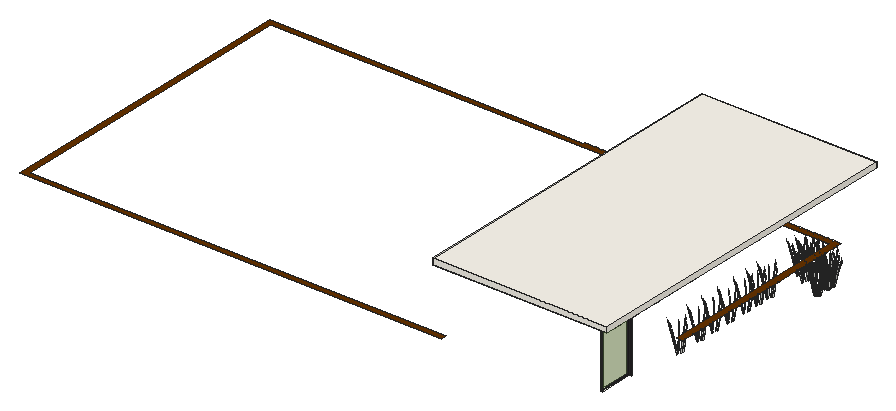
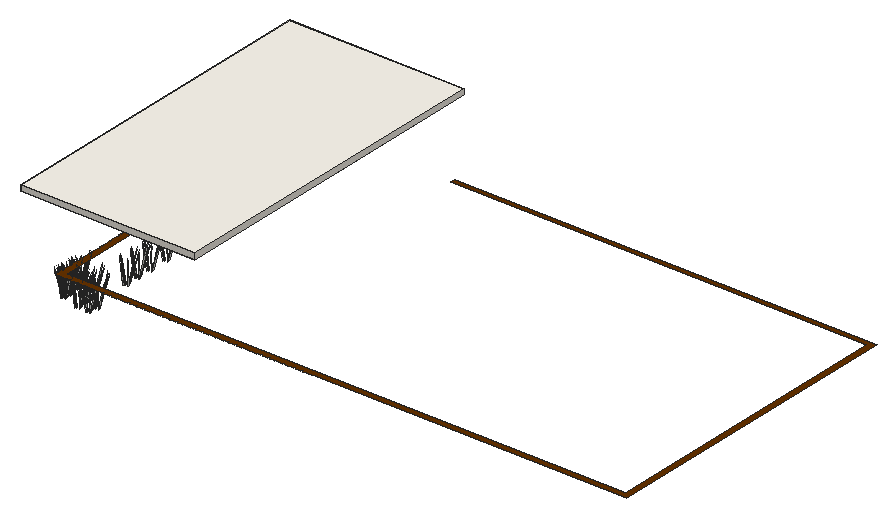
# SketchUp Ruby script. Lengths in inches.
U = 1.inch
M = Sketchup.active_model
def pt(a) = Geom::Point3d.new(a.map { |v| v * U })
def face(e, loops, mat)
  f = e.add_face(loops[0].map { |a| pt(a) })
  loops[1..].each { |l| e.add_face(l.map { |a| pt(a) }).erase! }
  f.material = f.back_material = mat if mat
  f
end
# faces: each face lists its corners as indices into pts; further lists are holes
def faces(e, pts, list, mat = nil) = list.each { |f| face(e, (f[0].is_a?(Array) ? f : [f]).map { |l| l.map { |i| pts[i] } }, mat) }
# xy, xz, yz: faces in a plane at the given z, y or x. An outline is a flat list of corners, or four numbers for a rectangle; further outlines are holes
def ring(l) = l.size == 4 ? [[l[0], l[1]], [l[2], l[1]], [l[2], l[3]], [l[0], l[3]]] : l.each_slice(2).to_a
def flat(e, list, mat, &to3) = list.each { |f| face(e, (f[0].is_a?(Array) ? f : [f]).map { |l| ring(l).map { |u, v| to3.(u, v) } }, mat) }
def xy(e, z, list, mat = nil) = flat(e, list, mat) { |x, y| [x, y, z] }
def xz(e, y, list, mat = nil) = flat(e, list, mat) { |x, z| [x, y, z] }
def yz(e, x, list, mat = nil) = flat(e, list, mat) { |y, z| [x, y, z] }
def lines(e, pts, list) = list.each { |a, b| e.add_line(pt(pts[a]), pt(pts[b])) }
# prism: a flat outline (further loops are holes) pulled along v
def prism(e, loops, v, mat = nil)
  f = face(e, loops, mat); d = Geom::Vector3d.new(v.map { |x| x * U })
  f.pushpull(f.normal.samedirection?(d) ? d.length : -d.length)
end
def box(e, o, s, mat = nil) = prism(e, [[o, [o[0] + s[0], o[1], o[2]], [o[0] + s[0], o[1] + s[1], o[2]], [o[0], o[1] + s[1], o[2]]]], [0, 0, s[2]], mat)
def at(x, y, z, deg = 0) = Geom::Transformation.translation(pt([x, y, z])) * Geom::Transformation.rotation(ORIGIN, Z_AXIS, deg.degrees)
def axes(o, x, y, z) = Geom::Transformation.new([*x, 0, *y, 0, *z, 0, *pt(o).to_a, 1])
def part(name) = M.definitions.add(name)
# library, detail: a bought-in or finely detailed component or shape, given as its bounding box
def library(name, o, s) = part(name).tap { |d| box(d.entities, o, s) }
def detail(e, o, s) = box(e.add_group.entities, o, s)
def put(e, d, t, mat = nil) = e.add_instance(d, t).tap { |i| i.material = mat if mat }
def group(e, t, mat = nil) = e.add_group.tap { |g| g.transformation = t; g.material = mat if mat }.entities
root = M.entities
M.materials.add("B04_Peach_Ember").color = [234, 141, 54]
M.materials.add("C01_Vanilla_Cream").color = [255, 251, 241]
M.materials.add("C08_Toffee_Ember").color = [102, 51, 0]
M.materials.add("Glass_Basic_01").color = [119, 186, 61]
M.materials["Glass_Basic_01"].alpha = 0.25
M.materials.add("LightPink_Translucent").color = [144, 107, 117]
M.materials["LightPink_Translucent"].alpha = 0.75
M.materials.add("Marble_07_1K").color = [36, 34, 36]
c1 = part("blade")
p = [[2.15,0.21,22],[0,0.17,0],[0.09,0.45,0],[2.18,0.31,22],[2.29,0.31,22],[0.38,0.45,0],
  [2.48,0.24,33],[2.49,0.24,33],[2.48,0.22,33]]
faces(c1.entities,p,[[0,1,2,3],[4,5,2,3],[6,3,4,7],[8,0,3,6]])
c2 = part("seeds")
p = [[0.3,-0.1,1.38],[-0.01,-0.03,1.59],[-0.01,-0.03,0.03],[0.14,-0.07,-0.07],[0.29,-0.03,3],[0.15,0.01,3.11]]
faces(c2.entities,p,[[0,1,2,3],[1,0,4,5]],"LightPink_Translucent")
c3 = part("blade with seeds")
put(c3.entities,c1,at(0,0,0))
put(c3.entities,c2,axes([2.4,0.25,30.99],[1.5799,-0.05474,1.17369],[-0.12525,1.92788,0.29478],[-0.07173,-0.02425,1.56792]))
xy(root,546,[[69,18,531,18,531,24,75,24,75,354,687.41,354,687.41,144,694.41,144,694.41,146.7,693.41,146.7,693.41,149.4,694.41,149.4,694.41,152.1,693.41,152.1,693.41,154.8,694.41,154.8,694.41,157.5,693.41,157.5,693.41,160.2,694.41,160.2,694.41,162.9,693.41,162.9,693.41,165.6,694.41,165.6,694.41,168.3,693.41,168.3,693.41,171,694.41,171,694.41,173.7,693.41,173.7,693.41,176.4,694.41,176.4,694.41,179.1,693.41,179.1,693.41,181.8,694.41,181.8,694.41,184.5,693.41,184.5,693.41,187.2,694.41,187.2,694.41,189.9,693.41,189.9,693.41,192.6,694.41,192.6,694.41,195.3,693.41,195.3,693.41,198,694.41,198,694.41,200.7,693.41,200.7,693.41,203.4,694.41,203.4,694.41,206.1,693.41,206.1,693.41,208.8,694.41,208.8,694.41,211.5,693.41,211.5,693.41,214.2,694.41,214.2,694.41,219.6,693.41,219.6,693.41,222.3,694.41,222.3,694.41,225,693.41,225,693.41,227.7,694.41,227.7,694.41,230.4,693.41,230.4,693.41,233.1,694.41,233.1,694.41,235.8,693.41,235.8,693.41,238.5,694.41,238.5,694.41,241.2,693.41,241.2,693.41,243.9,694.41,243.9,694.41,246.6,693.41,246.6,693.41,249.3,694.41,249.3,694.41,252,693.41,252,693.41,254.7,694.41,254.7,694.41,257.4,693.41,257.4,693.41,260.1,694.41,260.1,694.41,262.8,693.41,262.8,693.41,265.5,694.41,265.5,694.41,268.2,693.41,268.2,693.41,270.9,694.41,270.9,694.41,273.6,693.41,273.6,693.41,276.3,694.41,276.3,694.41,279,693.41,279,693.41,281.7,694.41,281.7,694.41,284.4,693.41,284.4,693.41,287.1,694.41,287.1,694.41,289.8,693.41,289.8,693.41,292.5,694.41,292.5,694.41,295.2,693.41,295.2,693.41,297.9,694.41,297.9,694.41,300.6,693.41,300.6,693.41,303.3,694.41,303.3,694.41,306,693.41,306,693.41,308.7,694.41,308.7,694.41,311.4,693.41,311.4,693.41,314.1,694.41,314.1,694.41,316.8,693.41,316.8,693.41,319.5,694.41,319.5,694.41,322.2,693.41,322.2,693.41,324.9,694.41,324.9,694.41,327.6,693.41,327.6,693.41,330.3,694.41,330.3,694.41,333,693.41,333,693.41,335.7,694.41,335.7,694.41,338.4,693.41,338.4,693.41,341.1,694.41,341.1,694.41,343.8,693.41,343.8,693.41,346.5,694.41,346.5,694.41,349.2,693.41,349.2,693.41,351.9,694.41,351.9,694.41,354.6,693.41,354.6,693.41,357.3,694.41,357.3,694.41,361,691.4,361,691.4,360,689.38,360,689.38,361,687.36,361,687.36,360,685.34,360,685.34,361,683.33,361,683.33,360,681.31,360,681.31,361,679.29,361,679.29,360,677.28,360,677.28,361,675.26,361,675.26,360,673.24,360,673.24,361,671.22,361,671.22,360,669.21,360,669.21,361,667.1875,361,667.1875,360,665.17,360,665.17,361,663.15,361,663.15,360,661.14,360,661.14,361,659.12,361,659.12,360,657.1,360,657.1,361,655.09,361,655.09,360,653.07,360,653.07,361,651.05,361,651.05,360,649.03,360,649.03,361,647.02,361,647.02,360,645,360,645,361,642.98,361,642.98,360,640.97,360,640.97,361.13,638.95,361.13,638.95,360,636.93,360,636.93,361.13,634.91,361.13,634.91,360,632.9,360,632.9,361.13,630.88,361.13,630.88,360,628.86,360,628.86,361.13,626.84,361.13,626.84,360,624.83,360,624.83,361.13,622.81,361.13,622.81,360,620.79,360,620.79,361.13,618.78,361.13,618.78,360,616.76,360,616.76,361.13,614.74,361.13,614.74,360,612.72,360,612.72,361.13,610.71,361.13,610.71,360,608.6875,360,608.6875,361.13,606.67,361.13,606.67,360,604.65,360,604.65,361.13,602.64,361.13,602.64,360,600.62,360,600.62,361.13,598.6,361.13,598.6,360,596.59,360,596.59,361.1875,594.57,361.1875,594.57,360,592.55,360,592.55,361.1875,590.53,361.1875,590.53,360,588.52,360,588.52,361.1875,586.5,361.1875,586.5,360,584.48,360,584.48,361.1875,582.47,361.1875,582.47,360,580.45,360,580.45,361.1875,578.43,361.1875,578.43,360,576.41,360,576.41,361.1875,574.4,361.1875,574.4,360,572.38,360,572.38,361.1875,570.36,361.1875,570.36,360,568.34,360,568.34,361.1875,566.33,361.1875,566.33,360,564.31,360,564.31,361.1875,562.29,361.1875,562.29,360,560.28,360,560.28,361.1875,558.26,361.1875,558.26,360,556.24,360,556.24,361.1875,554.22,361.1875,554.22,360,552.21,360,552.21,361.1875,550.1875,361.1875,550.1875,360,548.17,360,548.17,361.1875,546.15,361.1875,546.15,360,544.14,360,544.14,361.1875,542.12,361.1875,542.12,360,540.1,360,540.1,361.1875,538.09,361.1875,538.09,360,536.07,360,536.07,361.1875,534.05,361.1875,534.05,360,532.03,360,532.03,361.1875,530.02,361.1875,530.02,360,528,360,528,361.1875,525.98,361.1875,525.98,360,523.97,360,523.97,361.1875,521.95,361.1875,521.95,360,519.93,360,519.93,361.1875,517.91,361.1875,517.91,360,515.9,360,515.9,361.1875,513.88,361.1875,513.88,360,511.86,360,511.86,361.1875,509.84,361.1875,509.84,360,507.83,360,507.83,361.1875,505.81,361.1875,505.81,360,503.79,360,503.79,361.1875,501.78,361.1875,501.78,360,499.76,360,499.76,361.1875,497.74,361.1875,497.74,360,495.72,360,495.72,361.1875,493.71,361.1875,493.71,360,491.69,360,491.69,361.1875,489.67,361.1875,489.67,360,487.66,360,487.66,361.1875,485.64,361.1875,485.64,360,483.62,360,483.62,361.1875,481.6,361.1875,481.6,360,479.59,360,479.59,361.1875,477.57,361.1875,477.57,360,475.55,360,475.55,361.1875,473.53,361.1875,473.53,360,471.52,360,471.52,361.09,469.5,361.09,469.5,360,467.48,360,467.48,361.09,465.47,361.09,465.47,360,463.45,360,463.45,361.09,461.43,361.09,461.43,360,459.41,360,459.41,361.09,457.4,361.09,457.4,360,455.38,360,455.38,361.09,453.36,361.09,453.36,360,451.34,360,451.34,361.09,449.33,361.09,449.33,360,447.31,360,447.31,361.09,445.29,361.09,445.29,360,443.28,360,443.28,361.09,441.26,361.09,441.26,360,439.24,360,439.24,361.09,437.22,361.09,437.22,360,435.21,360,435.21,361.09,433.19,361.09,433.19,360,431.17,360,431.17,361.09,429.16,361.09,429.16,360,427.14,360,427.14,361.11,425.12,361.11,425.12,360,423.1,360,423.1,361.11,421.09,361.11,421.09,360,419.07,360,419.07,361.11,417.05,361.11,417.05,360,415.03,360,415.03,361.11,413.02,361.11,413.02,360,69,360]],"C08_Toffee_Ember")
xy(root,551,[[700,25,702,59]],"C01_Vanilla_Cream")
xy(root,553,[[700,25,702,59]],"C01_Vanilla_Cream")
xy(root,615,[[700,72,706,180],[621.41,144,700,180]],"Marble_07_1K")
xy(root,623,[[700,25,702,59]],"C01_Vanilla_Cream")
xy(root,624,[[[531,6,722,6,722,24,702,24,702,60,706,60,706,180,531,180],[535,12,535,174,615.41,174,615.41,138,693.41,138,693.41,12]]],"C01_Vanilla_Cream")
xz(root,25,[[700,553,702,623]],"C01_Vanilla_Cream")
xz(root,59,[[700,553,702,623]],"C01_Vanilla_Cream")
xz(root,60,[[702,552,706,624]],"Marble_07_1K")
xz(root,180,[[621.41,615,706,624]],"Marble_07_1K")
yz(root,700,[[25,553,59,623]],"C01_Vanilla_Cream")
yz(root,702,[[25,553,59,623]],"Glass_Basic_01")
yz(root,702,[[[24,552,60,624],[25,553,59,623]]],"Marble_07_1K")
yz(root,706,[[72,615,180,624]],"Marble_07_1K")
p = [[700.48,205.24,625.23],[701.21,205.2,625.22],[701.52,205.18,625.22],[702.54,205.39,625.26],[703.47,205.86,625.36],[704.25,206.54,625.5],
  [704.82,207.4,625.68],[705.14,208.37,625.88],[705.18,209.09,626.03],[705.19,209.39,626.1],[704.98,210.39,626.31],[704.5,211.3,626.5],
  [703.81,212.0625,626.65],[702.93,212.62,626.77],[701.9375,212.9375,626.84],[701.21,212.97,626.84],[700.89,212.99,626.85],[699.87,212.78,626.8],
  [698.94,212.31,626.71],[698.17,211.63,626.5625],[697.6,210.77,626.39],[697.27,209.8,626.18],[697.24,209.09,626.03],[697.22,208.78,625.97],
  [697.4375,207.78,625.76],[697.91,206.87,625.57],[698.61,206.11,625.41],[699.48,205.55,625.3],[700.17,327.13,626.82],[701.21,327,626.85],
  [702.24,327.13,626.82],[703.21,327.52,626.74],[704.04,328.14,626.61],[704.67,328.96,626.44],[705.07,329.9,626.24],[705.21,330.91,626.03],
  [705.07,331.93,625.82],[704.67,332.87,625.625],[704.04,333.68,625.46],[703.21,334.3,625.33],[702.24,334.7,625.25],[701.21,334.83,625.22],
  [700.17,334.7,625.25],[699.21,334.3,625.33],[698.38,333.68,625.46],[697.74,332.87,625.625],[697.34,331.93,625.82],[697.21,330.91,626.03],
  [697.34,329.9,626.24],[697.74,328.96,626.44],[698.38,328.14,626.61],[699.21,327.52,626.74],[698,355.22,624],[553,355.22,624]]
faces(root,p,[[0,1,2,3,4,5,6,7,8,9,10,11,12,13,14,15,16,17,18,19,20,21,22,23,24,25,26,27],[28,29,30,31,32,33,34,35,36,37,38,39,40,41,42,43,44,45,46,47,48,49,50,51]],"C01_Vanilla_Cream")
lines(root,p,[[52,53]])
put(root,c3,axes([668.04,339.8125,514.19],[-0.56631,0.0816,0.29394],[-0.14954,-0.46647,-0.37948],[0.16229,-0.12529,0.72609]))
put(root,c3,axes([662.91,340.08,514.19],[0.54068,0.15928,0.29394],[-0.1577,0.46469,-0.37948],[-0.21769,0.04261,0.72609]))
put(root,c3,axes([667.27,338.88,514.19],[-0.4402,0.30062,0.29394],[-0.41671,-0.34326,-0.37948],[0.0634,-0.1744,0.72609]))
put(root,c3,axes([664.67,338.46,514.19],[0.10048,0.4599,0.29394],[-0.5744,0.12144,-0.37948],[-0.15428,-0.13179,0.72609]))
put(root,c3,axes([698.79,344.84,514.19],[0.19614,-0.43908,0.29394],[0.57222,0.12807,-0.37948],[0.05247,0.17678,0.72609]))
put(root,c3,axes([699.83,340.6,514.19],[-0.19614,0.43908,0.29394],[-0.57222,-0.12807,-0.37948],[-0.05247,-0.17678,0.72609]))
put(root,c3,axes([701.31,344.14,514.19],[-0.37017,-0.35748,0.29394],[0.42268,-0.3384,-0.37948],[0.21476,0.05149,0.72609]))
put(root,c3,axes([701.91,343.14,514.19],[-0.54068,-0.15928,0.29394],[0.1577,-0.46469,-0.37948],[0.21769,-0.04261,0.72609]))
put(root,c3,axes([697.31,341.29,514.19],[0.37017,0.35748,0.29394],[-0.42268,0.3384,-0.37948],[-0.21476,-0.05149,0.72609]))
put(root,c3,axes([697.55,344.34,514.19],[0.4402,-0.30062,0.29394],[0.41671,0.34326,-0.37948],[-0.0634,0.1744,0.72609]))
put(root,c3,axes([696.79,343.41,514.19],[0.56631,-0.0816,0.29394],[0.14954,0.46647,-0.37948],[-0.16229,0.12529,0.72609]))
put(root,c3,axes([700.16,344.76,514.19],[-0.10048,-0.4599,0.29394],[0.5744,-0.12144,-0.37948],[0.15428,0.13179,0.72609]))
put(root,c3,axes([701.82,342.02,514.19],[-0.56631,0.0816,0.29394],[-0.14954,-0.46647,-0.37948],[0.16229,-0.12529,0.72609]))
put(root,c3,axes([696.7,342.3,514.19],[0.54068,0.15928,0.29394],[-0.1577,0.46469,-0.37948],[-0.21769,0.04261,0.72609]))
put(root,c3,axes([701.06,341.1,514.19],[-0.4402,0.30062,0.29394],[-0.41671,-0.34326,-0.37948],[0.0634,-0.1744,0.72609]))
put(root,c3,axes([698.45,340.67,514.19],[0.10048,0.4599,0.29394],[-0.5744,0.12144,-0.37948],[-0.15428,-0.13179,0.72609]))
put(root,c3,axes([698.79,338.4375,514.19],[0.19614,-0.43908,0.29394],[0.57222,0.12807,-0.37948],[0.05247,0.17678,0.72609]))
put(root,c3,axes([699.83,334.2,514.19],[-0.19614,0.43908,0.29394],[-0.57222,-0.12807,-0.37948],[-0.05247,-0.17678,0.72609]))
put(root,c3,axes([701.31,337.74,514.19],[-0.37017,-0.35748,0.29394],[0.42268,-0.3384,-0.37948],[0.21476,0.05149,0.72609]))
put(root,c3,axes([701.91,336.74,514.19],[-0.54068,-0.15928,0.29394],[0.1577,-0.46469,-0.37948],[0.21769,-0.04261,0.72609]))
put(root,c3,axes([697.31,334.89,514.19],[0.37017,0.35748,0.29394],[-0.42268,0.3384,-0.37948],[-0.21476,-0.05149,0.72609]))
put(root,c3,axes([697.55,337.94,514.19],[0.4402,-0.30062,0.29394],[0.41671,0.34326,-0.37948],[-0.0634,0.1744,0.72609]))
put(root,c3,axes([696.79,337.01,514.19],[0.56631,-0.0816,0.29394],[0.14954,0.46647,-0.37948],[-0.16229,0.12529,0.72609]))
put(root,c3,axes([700.16,338.36,514.19],[-0.10048,-0.4599,0.29394],[0.5744,-0.12144,-0.37948],[0.15428,0.13179,0.72609]))
put(root,c3,axes([701.82,335.625,514.19],[-0.56631,0.0816,0.29394],[-0.14954,-0.46647,-0.37948],[0.16229,-0.12529,0.72609]))
put(root,c3,axes([696.7,335.9,514.19],[0.54068,0.15928,0.29394],[-0.1577,0.46469,-0.37948],[-0.21769,0.04261,0.72609]))
put(root,c3,axes([701.06,334.7,514.19],[-0.4402,0.30062,0.29394],[-0.41671,-0.34326,-0.37948],[0.0634,-0.1744,0.72609]))
put(root,c3,axes([698.45,334.27,514.19],[0.10048,0.4599,0.29394],[-0.5744,0.12144,-0.37948],[-0.15428,-0.13179,0.72609]))
put(root,c3,axes([698.79,324.9375,514.19],[0.19614,-0.43908,0.29394],[0.57222,0.12807,-0.37948],[0.05247,0.17678,0.72609]))
put(root,c3,axes([699.83,320.7,514.19],[-0.19614,0.43908,0.29394],[-0.57222,-0.12807,-0.37948],[-0.05247,-0.17678,0.72609]))
put(root,c3,axes([701.31,324.24,514.19],[-0.37017,-0.35748,0.29394],[0.42268,-0.3384,-0.37948],[0.21476,0.05149,0.72609]))
put(root,c3,axes([701.91,323.24,514.19],[-0.54068,-0.15928,0.29394],[0.1577,-0.46469,-0.37948],[0.21769,-0.04261,0.72609]))
put(root,c3,axes([697.31,321.39,514.19],[0.37017,0.35748,0.29394],[-0.42268,0.3384,-0.37948],[-0.21476,-0.05149,0.72609]))
put(root,c3,axes([697.55,324.44,514.19],[0.4402,-0.30062,0.29394],[0.41671,0.34326,-0.37948],[-0.0634,0.1744,0.72609]))
put(root,c3,axes([696.79,323.51,514.19],[0.56631,-0.0816,0.29394],[0.14954,0.46647,-0.37948],[-0.16229,0.12529,0.72609]))
put(root,c3,axes([700.16,324.86,514.19],[-0.10048,-0.4599,0.29394],[0.5744,-0.12144,-0.37948],[0.15428,0.13179,0.72609]))
put(root,c3,axes([701.82,322.125,514.19],[-0.56631,0.0816,0.29394],[-0.14954,-0.46647,-0.37948],[0.16229,-0.12529,0.72609]))
put(root,c3,axes([696.7,322.4,514.19],[0.54068,0.15928,0.29394],[-0.1577,0.46469,-0.37948],[-0.21769,0.04261,0.72609]))
put(root,c3,axes([701.06,321.2,514.19],[-0.4402,0.30062,0.29394],[-0.41671,-0.34326,-0.37948],[0.0634,-0.1744,0.72609]))
put(root,c3,axes([698.45,320.77,514.19],[0.10048,0.4599,0.29394],[-0.5744,0.12144,-0.37948],[-0.15428,-0.13179,0.72609]))
put(root,c3,axes([671.18,171.12,514.2],[-0.64106,-0.14927,0.44225],[0.21921,-0.49074,0.36465],[0.03852,0.19299,0.91512]))
put(root,c3,axes([671.18,198.58,514.2],[-0.64106,-0.14927,0.44225],[0.21921,-0.49074,0.36465],[0.03852,0.19299,0.91512]))
put(root,c3,axes([671.18,218.87,514.2],[-0.64106,-0.14927,0.44225],[0.21921,-0.49074,0.36465],[0.03852,0.19299,0.91512]))
put(root,c3,axes([671.18,240.57,514.2],[-0.64106,-0.14927,0.44225],[0.21921,-0.49074,0.36465],[0.03852,0.19299,0.91512]))
put(root,c3,axes([671.18,262.41,514.2],[-0.64106,-0.14927,0.44225],[0.21921,-0.49074,0.36465],[0.03852,0.19299,0.91512]))
put(root,c3,axes([671.18,279.27,514.2],[-0.64106,-0.14927,0.44225],[0.21921,-0.49074,0.36465],[0.03852,0.19299,0.91512]))
put(root,c3,axes([671.18,294.61,514.2],[-0.64106,-0.14927,0.44225],[0.21921,-0.49074,0.36465],[0.03852,0.19299,0.91512]))
put(root,c3,axes([678.56,351.53,514.2],[-0.64106,-0.14927,0.44225],[0.21921,-0.49074,0.36465],[0.03852,0.19299,0.91512]))
put(root,c3,axes([677.61,345.2,514.2],[-0.64106,-0.14927,0.44225],[0.21921,-0.49074,0.36465],[0.03852,0.19299,0.91512]))
put(root,c3,axes([676.62,335.52,514.2],[-0.64106,-0.14927,0.44225],[0.21921,-0.49074,0.36465],[0.03852,0.19299,0.91512]))
put(root,c3,axes([667.25,351.33,514.2],[-0.64106,-0.14927,0.44225],[0.21921,-0.49074,0.36465],[0.03852,0.19299,0.91512]))
put(root,c3,axes([664.99,342.98,514.2],[-0.64106,-0.14927,0.44225],[0.21921,-0.49074,0.36465],[0.03852,0.19299,0.91512]))
put(root,c3,axes([698.78,345.2,514.2],[-0.64106,-0.14927,0.44225],[0.21921,-0.49074,0.36465],[0.03852,0.19299,0.91512]))
put(root,c3,axes([698.78,338.8,514.2],[-0.64106,-0.14927,0.44225],[0.21921,-0.49074,0.36465],[0.03852,0.19299,0.91512]))
put(root,c3,axes([698.78,325.3,514.2],[-0.64106,-0.14927,0.44225],[0.21921,-0.49074,0.36465],[0.03852,0.19299,0.91512]))
put(root,c3,axes([669.12,166.9,514.23],[0.53728,-0.42137,0.44623],[0.46337,0.44748,0.36794],[-0.25207,-0.07773,0.92337]))
put(root,c3,axes([670.59,166.06,514.23],[0.72473,-0.14676,0.44623],[0.12578,0.57568,0.36794],[-0.17045,-0.16967,0.92337]))
put(root,c3,axes([669.12,194.35,514.23],[0.53728,-0.42137,0.44623],[0.46337,0.44748,0.36794],[-0.25207,-0.07773,0.92337]))
put(root,c3,axes([670.59,193.51,514.23],[0.72473,-0.14676,0.44623],[0.12578,0.57568,0.36794],[-0.17045,-0.16967,0.92337]))
put(root,c3,axes([669.12,214.65,514.23],[0.53728,-0.42137,0.44623],[0.46337,0.44748,0.36794],[-0.25207,-0.07773,0.92337]))
put(root,c3,axes([670.59,213.8,514.23],[0.72473,-0.14676,0.44623],[0.12578,0.57568,0.36794],[-0.17045,-0.16967,0.92337]))
put(root,c3,axes([669.12,236.34,514.23],[0.53728,-0.42137,0.44623],[0.46337,0.44748,0.36794],[-0.25207,-0.07773,0.92337]))
put(root,c3,axes([670.59,235.5,514.23],[0.72473,-0.14676,0.44623],[0.12578,0.57568,0.36794],[-0.17045,-0.16967,0.92337]))
put(root,c3,axes([669.12,258.1875,514.23],[0.53728,-0.42137,0.44623],[0.46337,0.44748,0.36794],[-0.25207,-0.07773,0.92337]))
put(root,c3,axes([670.59,257.35,514.23],[0.72473,-0.14676,0.44623],[0.12578,0.57568,0.36794],[-0.17045,-0.16967,0.92337]))
put(root,c3,axes([669.12,275.05,514.23],[0.53728,-0.42137,0.44623],[0.46337,0.44748,0.36794],[-0.25207,-0.07773,0.92337]))
put(root,c3,axes([670.59,274.21,514.23],[0.72473,-0.14676,0.44623],[0.12578,0.57568,0.36794],[-0.17045,-0.16967,0.92337]))
put(root,c3,axes([669.12,290.38,514.23],[0.53728,-0.42137,0.44623],[0.46337,0.44748,0.36794],[-0.25207,-0.07773,0.92337]))
put(root,c3,axes([670.59,289.54,514.23],[0.72473,-0.14676,0.44623],[0.12578,0.57568,0.36794],[-0.17045,-0.16967,0.92337]))
put(root,c3,axes([676.51,347.31,514.23],[0.53728,-0.42137,0.44623],[0.46337,0.44748,0.36794],[-0.25207,-0.07773,0.92337]))
put(root,c3,axes([677.97,346.46,514.23],[0.72473,-0.14676,0.44623],[0.12578,0.57568,0.36794],[-0.17045,-0.16967,0.92337]))
put(root,c3,axes([675.55,340.97,514.23],[0.53728,-0.42137,0.44623],[0.46337,0.44748,0.36794],[-0.25207,-0.07773,0.92337]))
put(root,c3,axes([677.02,340.13,514.23],[0.72473,-0.14676,0.44623],[0.12578,0.57568,0.36794],[-0.17045,-0.16967,0.92337]))
put(root,c3,axes([674.57,331.3,514.23],[0.53728,-0.42137,0.44623],[0.46337,0.44748,0.36794],[-0.25207,-0.07773,0.92337]))
put(root,c3,axes([676.03,330.46,514.23],[0.72473,-0.14676,0.44623],[0.12578,0.57568,0.36794],[-0.17045,-0.16967,0.92337]))
put(root,c3,axes([665.2,347.1,514.23],[0.53728,-0.42137,0.44623],[0.46337,0.44748,0.36794],[-0.25207,-0.07773,0.92337]))
put(root,c3,axes([666.66,346.26,514.23],[0.72473,-0.14676,0.44623],[0.12578,0.57568,0.36794],[-0.17045,-0.16967,0.92337]))
put(root,c3,axes([662.94,338.76,514.23],[0.53728,-0.42137,0.44623],[0.46337,0.44748,0.36794],[-0.25207,-0.07773,0.92337]))
put(root,c3,axes([664.41,337.92,514.23],[0.72473,-0.14676,0.44623],[0.12578,0.57568,0.36794],[-0.17045,-0.16967,0.92337]))
put(root,c3,axes([696.73,340.97,514.23],[0.53728,-0.42137,0.44623],[0.46337,0.44748,0.36794],[-0.25207,-0.07773,0.92337]))
put(root,c3,axes([698.19,340.13,514.23],[0.72473,-0.14676,0.44623],[0.12578,0.57568,0.36794],[-0.17045,-0.16967,0.92337]))
put(root,c3,axes([696.73,334.57,514.23],[0.53728,-0.42137,0.44623],[0.46337,0.44748,0.36794],[-0.25207,-0.07773,0.92337]))
put(root,c3,axes([698.19,333.73,514.23],[0.72473,-0.14676,0.44623],[0.12578,0.57568,0.36794],[-0.17045,-0.16967,0.92337]))
put(root,c3,axes([696.73,321.07,514.23],[0.53728,-0.42137,0.44623],[0.46337,0.44748,0.36794],[-0.25207,-0.07773,0.92337]))
put(root,c3,axes([698.19,320.23,514.23],[0.72473,-0.14676,0.44623],[0.12578,0.57568,0.36794],[-0.17045,-0.16967,0.92337]))
put(root,c3,axes([671.95,172.33,514.6875],[0.44958,-0.32756,-0.05385],[0.41194,0.35875,-0.24415],[0.029,0.10165,0.8053]))
put(root,c3,axes([667.9,170.66,514.6875],[0.5741,0.15241,-0.05385],[-0.1766,0.46909,-0.24415],[-0.0939,0.07122,0.8053]))
put(root,c3,axes([671.95,199.78,514.6875],[0.44958,-0.32756,-0.05385],[0.41194,0.35875,-0.24415],[0.029,0.10165,0.8053]))
put(root,c3,axes([667.9,198.12,514.6875],[0.5741,0.15241,-0.05385],[-0.1766,0.46909,-0.24415],[-0.0939,0.07122,0.8053]))
put(root,c3,axes([671.95,220.08,514.6875],[0.44958,-0.32756,-0.05385],[0.41194,0.35875,-0.24415],[0.029,0.10165,0.8053]))
put(root,c3,axes([667.9,218.41,514.6875],[0.5741,0.15241,-0.05385],[-0.1766,0.46909,-0.24415],[-0.0939,0.07122,0.8053]))
put(root,c3,axes([671.95,241.77,514.6875],[0.44958,-0.32756,-0.05385],[0.41194,0.35875,-0.24415],[0.029,0.10165,0.8053]))
put(root,c3,axes([667.9,240.11,514.6875],[0.5741,0.15241,-0.05385],[-0.1766,0.46909,-0.24415],[-0.0939,0.07122,0.8053]))
put(root,c3,axes([671.95,263.62,514.6875],[0.44958,-0.32756,-0.05385],[0.41194,0.35875,-0.24415],[0.029,0.10165,0.8053]))
put(root,c3,axes([667.9,261.95,514.6875],[0.5741,0.15241,-0.05385],[-0.1766,0.46909,-0.24415],[-0.0939,0.07122,0.8053]))
put(root,c3,axes([671.95,280.48,514.6875],[0.44958,-0.32756,-0.05385],[0.41194,0.35875,-0.24415],[0.029,0.10165,0.8053]))
put(root,c3,axes([667.9,278.8125,514.6875],[0.5741,0.15241,-0.05385],[-0.1766,0.46909,-0.24415],[-0.0939,0.07122,0.8053]))
put(root,c3,axes([671.95,295.8125,514.6875],[0.44958,-0.32756,-0.05385],[0.41194,0.35875,-0.24415],[0.029,0.10165,0.8053]))
put(root,c3,axes([667.9,294.15,514.6875],[0.5741,0.15241,-0.05385],[-0.1766,0.46909,-0.24415],[-0.0939,0.07122,0.8053]))
put(root,c3,axes([679.34,352.73,514.6875],[0.44958,-0.32756,-0.05385],[0.41194,0.35875,-0.24415],[0.029,0.10165,0.8053]))
put(root,c3,axes([675.28,351.07,514.6875],[0.5741,0.15241,-0.05385],[-0.1766,0.46909,-0.24415],[-0.0939,0.07122,0.8053]))
put(root,c3,axes([678.39,346.4,514.6875],[0.44958,-0.32756,-0.05385],[0.41194,0.35875,-0.24415],[0.029,0.10165,0.8053]))
put(root,c3,axes([674.33,344.74,514.6875],[0.5741,0.15241,-0.05385],[-0.1766,0.46909,-0.24415],[-0.0939,0.07122,0.8053]))
put(root,c3,axes([677.4,336.73,514.6875],[0.44958,-0.32756,-0.05385],[0.41194,0.35875,-0.24415],[0.029,0.10165,0.8053]))
put(root,c3,axes([673.34,335.0625,514.6875],[0.5741,0.15241,-0.05385],[-0.1766,0.46909,-0.24415],[-0.0939,0.07122,0.8053]))
put(root,c3,axes([668.03,352.53,514.6875],[0.44958,-0.32756,-0.05385],[0.41194,0.35875,-0.24415],[0.029,0.10165,0.8053]))
put(root,c3,axes([663.97,350.87,514.6875],[0.5741,0.15241,-0.05385],[-0.1766,0.46909,-0.24415],[-0.0939,0.07122,0.8053]))
put(root,c3,axes([665.77,344.19,514.6875],[0.44958,-0.32756,-0.05385],[0.41194,0.35875,-0.24415],[0.029,0.10165,0.8053]))
put(root,c3,axes([661.72,342.52,514.6875],[0.5741,0.15241,-0.05385],[-0.1766,0.46909,-0.24415],[-0.0939,0.07122,0.8053]))
put(root,c3,axes([699.56,346.4,514.6875],[0.44958,-0.32756,-0.05385],[0.41194,0.35875,-0.24415],[0.029,0.10165,0.8053]))
put(root,c3,axes([695.5,344.74,514.6875],[0.5741,0.15241,-0.05385],[-0.1766,0.46909,-0.24415],[-0.0939,0.07122,0.8053]))
put(root,c3,axes([699.56,340,514.6875],[0.44958,-0.32756,-0.05385],[0.41194,0.35875,-0.24415],[0.029,0.10165,0.8053]))
put(root,c3,axes([695.5,338.34,514.6875],[0.5741,0.15241,-0.05385],[-0.1766,0.46909,-0.24415],[-0.0939,0.07122,0.8053]))
put(root,c3,axes([699.56,326.5,514.6875],[0.44958,-0.32756,-0.05385],[0.41194,0.35875,-0.24415],[0.029,0.10165,0.8053]))
put(root,c3,axes([695.5,324.84,514.6875],[0.5741,0.15241,-0.05385],[-0.1766,0.46909,-0.24415],[-0.0939,0.07122,0.8053]))
g1 = group(root,at(531,6,624),"C01_Vanilla_Cream")
xy(g1,-1,[[22,174.66,22,349.22,167,349.22,167,174.66,165.5,174.66,165.5,346.92,24,346.92,24,174.66]],"C08_Toffee_Ember")
xy(g1,0,[[0,0,0,174.66,191,174.66,191,174,175,174,175,18,191,18,191,0],[175,18,191,23.2],[175,28.4,191,33.6],[175,38.8,191,44],[175,49.2,191,54.4],
  [175,59.6,191,64.8],[175,70,191,75.2],[175,80.4,191,85.6],[175,90.8,191,96],[175,101.2,191,106.4],
  [175,111.6,191,116.8],[175,122,191,127.2],[175,132.4,191,137.6],[175,142.8,191,148],[175,153.2,191,158.4],
  [175,163.6,191,168.8],[0,174.66,22,179.51],[24,174.66,165.5,179.51],[167,174.66,191,179.51],[0,184.36,22,189.21],
  [24,184.36,165.5,189.21],[167,184.36,191,189.21],[0,194.06,22,198.9],[24,194.06,165.5,198.9],[167,194.06,191,198.9],
  [0,203.75,22,208.6],[24,203.75,165.5,208.6],[167,203.75,191,208.6],[0,213.45,22,218.3],[24,213.45,165.5,218.3],
  [167,213.45,191,218.3],[0,223.15,22,228],[24,223.15,165.5,228],[167,223.15,191,228],[0,232.85,22,237.7],
  [24,232.85,165.5,237.7],[167,232.85,191,237.7],[0,242.54,22,247.39],[24,242.54,165.5,247.39],[167,242.54,191,247.39],
  [0,252.24,22,257.09],[24,252.24,165.5,257.09],[167,252.24,191,257.09],[0,261.94,22,266.79],[24,261.94,165.5,266.79],
  [167,261.94,191,266.79],[0,271.64,22,276.49],[24,271.64,165.5,276.49],[167,271.64,191,276.49],[0,281.34,22,286.19],
  [24,281.34,165.5,286.19],[167,281.34,191,286.19],[0,291.03,22,295.88],[24,291.03,165.5,295.88],[167,291.03,191,295.88],
  [0,300.73,22,305.58],[24,300.73,165.5,305.58],[167,300.73,191,305.58],[0,310.43,22,315.28],[24,310.43,165.5,315.28],
  [167,310.43,191,315.28],[0,320.13,22,324.98],[24,320.13,165.5,324.98],[167,320.13,191,324.98],[0,329.83,22,334.68],
  [24,329.83,165.5,334.68],[167,329.83,191,334.68],[0,339.52,22,344.375],[24,339.52,165.5,344.375],[167,339.52,191,344.375],
  [0,349.22,191,354.07],[0,358.92,191,363.77]])
xy(g1,0,[[175,23.2,191,28.4],[175,33.6,191,38.8],[175,44,191,49.2],[175,54.4,191,59.6],[175,64.8,191,70],
  [175,75.2,191,80.4],[175,85.6,191,90.8],[175,96,191,101.2],[175,106.4,191,111.6],[175,116.8,191,122],
  [175,127.2,191,132.4],[175,137.6,191,142.8],[175,148,191,153.2],[175,158.4,191,163.6],[175,168.8,191,174],
  [0,179.51,22,184.36],[24,179.51,165.5,184.36],[167,179.51,191,184.36],[0,189.21,22,194.06],[24,189.21,165.5,194.06],
  [167,189.21,191,194.06],[0,198.9,22,203.75],[24,198.9,165.5,203.75],[167,198.9,191,203.75],[0,208.6,22,213.45],
  [24,208.6,165.5,213.45],[167,208.6,191,213.45],[0,218.3,22,223.15],[24,218.3,165.5,223.15],[167,218.3,191,223.15],
  [0,228,22,232.85],[24,228,165.5,232.85],[167,228,191,232.85],[0,237.7,22,242.54],[24,237.7,165.5,242.54],
  [167,237.7,191,242.54],[0,247.39,22,252.24],[24,247.39,165.5,252.24],[167,247.39,191,252.24],[0,257.09,22,261.94],
  [24,257.09,165.5,261.94],[167,257.09,191,261.94],[0,266.79,22,271.64],[24,266.79,165.5,271.64],[167,266.79,191,271.64],
  [0,276.49,22,281.34],[24,276.49,165.5,281.34],[167,276.49,191,281.34],[0,286.19,22,291.03],[24,286.19,165.5,291.03],
  [167,286.19,191,291.03],[0,295.88,22,300.73],[24,295.88,165.5,300.73],[167,295.88,191,300.73],[0,305.58,22,310.43],
  [24,305.58,165.5,310.43],[167,305.58,191,310.43],[0,315.28,22,320.13],[24,315.28,165.5,320.13],[167,315.28,191,320.13],
  [0,324.98,22,329.83],[24,324.98,165.5,329.83],[167,324.98,191,329.83],[0,334.68,22,339.52],[24,334.68,165.5,339.52],
  [167,334.68,191,339.52],[0,344.375,22,349.22],[24,344.375,165.5,346.92],[167,344.375,191,349.22],[0,354.07,191,358.92],
  [0,363.77,191,368.62]],"B04_Peach_Ember")
xy(g1,6,[[0,0,191,368.62]])
xz(g1,0,[[0,0,191,6]])
xz(g1,174.66,[[22,-1,24,0],[165.5,-1,167,0]],"B04_Peach_Ember")
xz(g1,346.92,[[24,-1,164,0],[164,-1,165.5,0]],"B04_Peach_Ember")
xz(g1,349.22,[[22,-1,167,0]],"B04_Peach_Ember")
xz(g1,368.62,[[0,0,191,6]])
yz(g1,0,[[0,0,368.62,6]])
yz(g1,22,[[174.66,-1,179.51,0],[179.51,-1,184.36,0],[184.36,-1,189.21,0],[189.21,-1,194.06,0],[194.06,-1,198.9,0],
  [198.9,-1,203.75,0],[203.75,-1,208.6,0],[208.6,-1,213.45,0],[213.45,-1,218.3,0],[218.3,-1,223.15,0],
  [223.15,-1,228,0],[228,-1,232.85,0],[232.85,-1,237.7,0],[237.7,-1,242.54,0],[242.54,-1,247.39,0],
  [247.39,-1,252.24,0],[252.24,-1,257.09,0],[257.09,-1,261.94,0],[261.94,-1,266.79,0],[266.79,-1,271.64,0],
  [271.64,-1,276.49,0],[276.49,-1,281.34,0],[281.34,-1,286.19,0],[286.19,-1,291.03,0],[291.03,-1,295.88,0],
  [295.88,-1,300.73,0],[300.73,-1,305.58,0],[305.58,-1,310.43,0],[310.43,-1,315.28,0],[315.28,-1,320.13,0],
  [320.13,-1,324.98,0],[324.98,-1,329.83,0],[329.83,-1,334.68,0],[334.68,-1,339.52,0],[339.52,-1,344.375,0],
  [344.375,-1,349.22,0]],"B04_Peach_Ember")
yz(g1,24,[[174.66,-1,179.51,0],[179.51,-1,184.36,0],[184.36,-1,189.21,0],[189.21,-1,194.06,0],[194.06,-1,198.9,0],
  [198.9,-1,203.75,0],[203.75,-1,208.6,0],[208.6,-1,213.45,0],[213.45,-1,218.3,0],[218.3,-1,223.15,0],
  [223.15,-1,228,0],[228,-1,232.85,0],[232.85,-1,237.7,0],[237.7,-1,242.54,0],[242.54,-1,247.39,0],
  [247.39,-1,252.24,0],[252.24,-1,257.09,0],[257.09,-1,261.94,0],[261.94,-1,266.79,0],[266.79,-1,271.64,0],
  [271.64,-1,276.49,0],[276.49,-1,281.34,0],[281.34,-1,286.19,0],[286.19,-1,291.03,0],[291.03,-1,295.88,0],
  [295.88,-1,300.73,0],[300.73,-1,305.58,0],[305.58,-1,310.43,0],[310.43,-1,315.28,0],[315.28,-1,320.13,0],
  [320.13,-1,324.98,0],[324.98,-1,329.83,0],[329.83,-1,334.68,0],[334.68,-1,339.52,0],[339.52,-1,344.375,0],
  [344.375,-1,346.92,0]],"B04_Peach_Ember")
yz(g1,165.5,[[174.66,-1,179.51,0],[179.51,-1,184.36,0],[184.36,-1,189.21,0],[189.21,-1,194.06,0],[194.06,-1,198.9,0],
  [198.9,-1,203.75,0],[203.75,-1,208.6,0],[208.6,-1,213.45,0],[213.45,-1,218.3,0],[218.3,-1,223.15,0],
  [223.15,-1,228,0],[228,-1,232.85,0],[232.85,-1,237.7,0],[237.7,-1,242.54,0],[242.54,-1,247.39,0],
  [247.39,-1,252.24,0],[252.24,-1,257.09,0],[257.09,-1,261.94,0],[261.94,-1,266.79,0],[266.79,-1,271.64,0],
  [271.64,-1,276.49,0],[276.49,-1,281.34,0],[281.34,-1,286.19,0],[286.19,-1,291.03,0],[291.03,-1,295.88,0],
  [295.88,-1,300.73,0],[300.73,-1,305.58,0],[305.58,-1,310.43,0],[310.43,-1,315.28,0],[315.28,-1,320.13,0],
  [320.13,-1,324.98,0],[324.98,-1,329.83,0],[329.83,-1,334.68,0],[334.68,-1,339.52,0],[339.52,-1,344.375,0],
  [344.375,-1,346.92,0]],"B04_Peach_Ember")
yz(g1,167,[[174.66,-1,179.51,0],[179.51,-1,184.36,0],[184.36,-1,189.21,0],[189.21,-1,194.06,0],[194.06,-1,198.9,0],
  [198.9,-1,203.75,0],[203.75,-1,208.6,0],[208.6,-1,213.45,0],[213.45,-1,218.3,0],[218.3,-1,223.15,0],
  [223.15,-1,228,0],[228,-1,232.85,0],[232.85,-1,237.7,0],[237.7,-1,242.54,0],[242.54,-1,247.39,0],
  [247.39,-1,252.24,0],[252.24,-1,257.09,0],[257.09,-1,261.94,0],[261.94,-1,266.79,0],[266.79,-1,271.64,0],
  [271.64,-1,276.49,0],[276.49,-1,281.34,0],[281.34,-1,286.19,0],[286.19,-1,291.03,0],[291.03,-1,295.88,0],
  [295.88,-1,300.73,0],[300.73,-1,305.58,0],[305.58,-1,310.43,0],[310.43,-1,315.28,0],[315.28,-1,320.13,0],
  [320.13,-1,324.98,0],[324.98,-1,329.83,0],[329.83,-1,334.68,0],[334.68,-1,339.52,0],[339.52,-1,344.375,0],
  [344.375,-1,349.22,0]],"B04_Peach_Ember")
yz(g1,191,[[0,0,368.62,6]])
p = [[24,174.66,0],[24,174,0],[22,174.66,0],[22,174,0]]
lines(g1,p,[[0,1],[2,3]])
